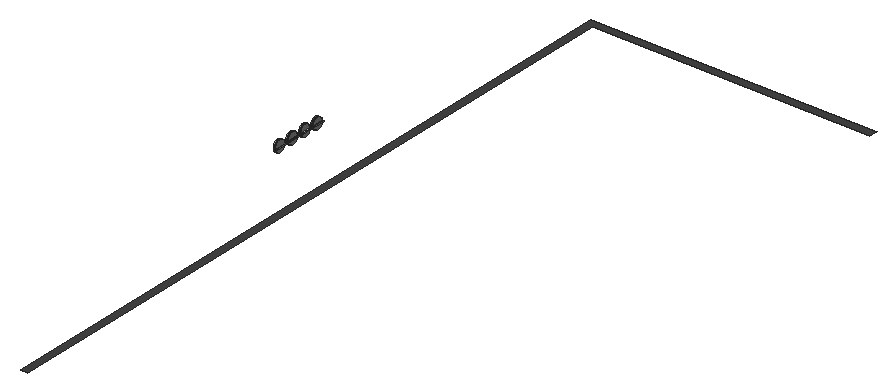
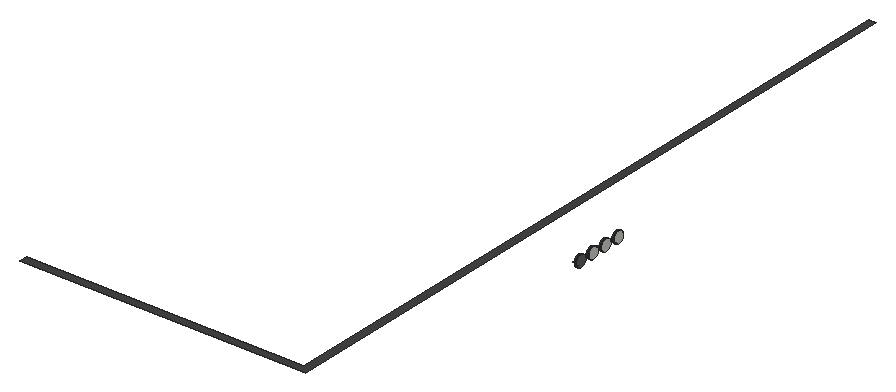
# SketchUp Ruby script. Lengths in inches.
U = 1.inch
M = Sketchup.active_model
def pt(a) = Geom::Point3d.new(a.map { |v| v * U })
def face(e, loops, mat)
  f = e.add_face(loops[0].map { |a| pt(a) })
  loops[1..].each { |l| e.add_face(l.map { |a| pt(a) }).erase! }
  f.material = f.back_material = mat if mat
  f
end
# faces: each face lists its corners as indices into pts; further lists are holes
def faces(e, pts, list, mat = nil) = list.each { |f| face(e, (f[0].is_a?(Array) ? f : [f]).map { |l| l.map { |i| pts[i] } }, mat) }
# xy, xz, yz: faces in a plane at the given z, y or x. An outline is a flat list of corners, or four numbers for a rectangle; further outlines are holes
def ring(l) = l.size == 4 ? [[l[0], l[1]], [l[2], l[1]], [l[2], l[3]], [l[0], l[3]]] : l.each_slice(2).to_a
def flat(e, list, mat, &to3) = list.each { |f| face(e, (f[0].is_a?(Array) ? f : [f]).map { |l| ring(l).map { |u, v| to3.(u, v) } }, mat) }
def xy(e, z, list, mat = nil) = flat(e, list, mat) { |x, y| [x, y, z] }
def xz(e, y, list, mat = nil) = flat(e, list, mat) { |x, z| [x, y, z] }
def yz(e, x, list, mat = nil) = flat(e, list, mat) { |y, z| [x, y, z] }
def lines(e, pts, list) = list.each { |a, b| e.add_line(pt(pts[a]), pt(pts[b])) }
# prism: a flat outline (further loops are holes) pulled along v
def prism(e, loops, v, mat = nil)
  f = face(e, loops, mat); d = Geom::Vector3d.new(v.map { |x| x * U })
  f.pushpull(f.normal.samedirection?(d) ? d.length : -d.length)
end
def box(e, o, s, mat = nil) = prism(e, [[o, [o[0] + s[0], o[1], o[2]], [o[0] + s[0], o[1] + s[1], o[2]], [o[0], o[1] + s[1], o[2]]]], [0, 0, s[2]], mat)
def at(x, y, z, deg = 0) = Geom::Transformation.translation(pt([x, y, z])) * Geom::Transformation.rotation(ORIGIN, Z_AXIS, deg.degrees)
def axes(o, x, y, z) = Geom::Transformation.new([*x, 0, *y, 0, *z, 0, *pt(o).to_a, 1])
def part(name) = M.definitions.add(name)
# library, detail: a bought-in or finely detailed component or shape, given as its bounding box
def library(name, o, s) = part(name).tap { |d| box(d.entities, o, s) }
def detail(e, o, s) = box(e.add_group.entities, o, s)
def put(e, d, t, mat = nil) = e.add_instance(d, t).tap { |i| i.material = mat if mat }
def group(e, t, mat = nil) = e.add_group.tap { |g| g.transformation = t; g.material = mat if mat }.entities
root = M.entities
M.materials.add("[0134_DimGray]").color = [105, 105, 105]
M.materials.add("[Granite Dark Gray]").color = [69, 68, 68]
xy(root,110.72,[[126.73,150.81,127.73,151.02],[126.73,156.81,127.73,157.02],[126.73,162.81,127.73,163.02]],"[0134_DimGray]")
xy(root,111,[[150,0,153,0,153,267,258,267,258,270,150,270]],"[Granite Dark Gray]")
xy(root,112.48,[[127.73,148.85,128.23,152.82],[127.73,154.85,128.23,158.82],[127.73,160.85,128.23,164.82]],"[0134_DimGray]")
xy(root,112.5,[[127.73,166.66,128.23,170.65]],"[0134_DimGray]")
xy(root,112.73,[[127.73,166.66,128.23,170.64]],"[0134_DimGray]")
xy(root,112.74,[[127.73,148.84,128.23,152.82],[127.73,154.84,128.23,158.82],[127.73,160.84,128.23,164.82]],"[0134_DimGray]")
xz(root,148.84,[[126.73,112.53,127.73,112.74],[127.73,112.53,128.23,112.74]],"[0134_DimGray]")
xz(root,152.82,[[127.73,112.48,128.23,112.74]],"[0134_DimGray]")
xz(root,154.84,[[126.73,112.53,127.73,112.74],[127.73,112.53,128.23,112.74]],"[0134_DimGray]")
xz(root,158.82,[[127.73,112.48,128.23,112.74]],"[0134_DimGray]")
xz(root,160.84,[[126.73,112.53,127.73,112.74],[127.73,112.53,128.23,112.74]],"[0134_DimGray]")
xz(root,164.82,[[127.73,112.48,128.23,112.74]])
xz(root,166.66,[[127.73,112.5,128.23,112.73]],"[0134_DimGray]")
xz(root,170.64,[[127.73,112.71,128.23,112.73]],"[0134_DimGray]")
yz(root,126.73,[[150.81,110.72,150.6,110.73,150.39,110.77,150.19,110.82,150,110.9,149.8125,111,149.64,111.11,149.48,111.25,149.33,111.4,149.2,111.5625,149.09,111.74,149,111.93,148.92,112.125,148.875,112.33,148.84,112.53,148.84,112.74,148.85,112.95,148.89,113.16,148.94,113.36,149.02,113.55,149.12,113.74,149.23,113.91,149.37,114.07,149.52,114.22,149.68,114.35,149.86,114.46,150.05,114.55,150.24,114.625,150.45,114.68,150.65,114.71,150.86,114.72,151.07,114.7,151.28,114.67,151.48,114.61,151.67,114.53,151.86,114.43,152.03,114.32,152.19,114.18,152.34,114.03,152.47,113.87,152.58,113.69,152.67,113.5,152.75,113.31,152.8,113.1,152.83,112.9,152.84,112.6875,152.82,112.48,152.79,112.27,152.73,112.07,152.65,111.875,152.55,111.69,152.4375,111.52,152.3,111.36,152.15,111.21,151.99,111.08,151.8125,110.97,151.625,110.875,151.43,110.8,151.22,110.75,151.02,110.72],[156.81,110.72,156.6,110.73,156.39,110.77,156.19,110.82,156,110.9,155.8125,111,155.64,111.11,155.48,111.25,155.33,111.4,155.2,111.5625,155.09,111.74,155,111.93,154.92,112.125,154.875,112.33,154.84,112.53,154.84,112.74,154.85,112.95,154.89,113.16,154.94,113.36,155.02,113.55,155.12,113.74,155.23,113.91,155.37,114.07,155.52,114.22,155.68,114.35,155.86,114.46,156.05,114.55,156.24,114.625,156.45,114.68,156.65,114.71,156.86,114.72,157.07,114.7,157.28,114.67,157.48,114.61,157.67,114.53,157.86,114.43,158.03,114.32,158.19,114.18,158.34,114.03,158.47,113.87,158.58,113.69,158.67,113.5,158.75,113.31,158.8,113.1,158.83,112.9,158.84,112.6875,158.82,112.48,158.79,112.27,158.73,112.07,158.65,111.875,158.55,111.69,158.4375,111.52,158.3,111.36,158.15,111.21,157.99,111.08,157.8125,110.97,157.625,110.875,157.43,110.8,157.22,110.75,157.02,110.72],[162.81,110.72,162.6,110.73,162.39,110.77,162.19,110.82,162,110.9,161.8125,111,161.64,111.11,161.48,111.25,161.33,111.4,161.2,111.5625,161.09,111.74,161,111.93,160.92,112.125,160.875,112.33,160.84,112.53,160.84,112.74,160.85,112.95,160.89,113.16,160.94,113.36,161.02,113.55,161.12,113.74,161.23,113.91,161.37,114.07,161.52,114.22,161.68,114.35,161.86,114.46,162.05,114.55,162.24,114.625,162.45,114.68,162.65,114.71,162.86,114.72,163.07,114.7,163.28,114.67,163.48,114.61,163.67,114.53,163.86,114.43,164.03,114.32,164.19,114.18,164.34,114.03,164.47,113.87,164.58,113.69,164.67,113.5,164.75,113.31,164.8,113.1,164.83,112.9,164.84,112.6875,164.82,112.48,164.79,112.27,164.73,112.07,164.65,111.875,164.55,111.69,164.4375,111.52,164.3,111.36,164.15,111.21,163.99,111.08,163.8125,110.97,163.625,110.875,163.43,110.8,163.22,110.75,163.02,110.72]])
yz(root,126.73,[[168.64,110.51,168.43,110.52,168.23,110.56,168.02,110.61,167.83,110.6875,167.64,110.79,167.47,110.9,167.31,111.03,167.16,111.18,167.03,111.34,166.91,111.52,166.82,111.71,166.75,111.9,166.69,112.11,166.66,112.3125,166.65,112.52,166.66,112.73,166.7,112.9375,166.75,113.14,166.83,113.33,166.92,113.52,167.04,113.7,167.17,113.86,167.32,114.01,167.48,114.14,167.66,114.25,167.85,114.34,168.04,114.42,168.25,114.47,168.45,114.5,168.66,114.51,168.87,114.5,169.08,114.47,169.28,114.41,169.47,114.34,169.66,114.24,169.84,114.125,170,113.99,170.14,113.84,170.28,113.68,170.39,113.5,170.48,113.32,170.56,113.12,170.61,112.92,170.64,112.71,170.65,112.5,170.64,112.29,170.61,112.09,170.55,111.89,170.47,111.69,170.38,111.5,170.26,111.33,170.13,111.17,169.98,111.02,169.82,110.89,169.64,110.78,169.46,110.68,169.26,110.61,169.06,110.55,168.85,110.52]],"[0134_DimGray]")
yz(root,127.73,[[148.84,112.48,148.85,112.48,148.84,112.53,148.84,112.74],[154.85,112.48,154.84,112.53,154.84,112.74,158.82,112.74,158.82,112.48],[160.85,112.48,160.84,112.53,160.84,112.74,164.82,112.74,164.82,112.48],[170.65,112.5,170.65,112.73,170.64,112.73,170.64,112.71]])
yz(root,127.73,[[168.64,110.51,168.85,110.52,169.06,110.55,169.26,110.61,169.46,110.68,169.64,110.78,169.82,110.89,169.98,111.02,170.13,111.17,170.26,111.33,170.38,111.5,170.47,111.69,170.55,111.89,170.61,112.09,170.64,112.29,170.65,112.5,166.66,112.5,166.66,112.73,166.65,112.52,166.66,112.3125,166.69,112.11,166.75,111.9,166.82,111.71,166.91,111.52,167.03,111.34,167.16,111.18,167.31,111.03,167.47,110.9,167.64,110.79,167.83,110.6875,168.02,110.61,168.23,110.56,168.43,110.52],[150.81,110.72,151.02,110.72,151.22,110.75,151.43,110.8,151.625,110.875,151.8125,110.97,151.99,111.08,152.15,111.21,152.3,111.36,152.4375,111.52,152.55,111.69,152.65,111.875,152.73,112.07,152.79,112.27,152.82,112.48,148.85,112.48,148.875,112.33,148.92,112.125,149,111.93,149.09,111.74,149.2,111.5625,149.33,111.4,149.48,111.25,149.64,111.11,149.8125,111,150,110.9,150.19,110.82,150.39,110.77,150.6,110.73],[156.81,110.72,157.02,110.72,157.22,110.75,157.43,110.8,157.625,110.875,157.8125,110.97,157.99,111.08,158.15,111.21,158.3,111.36,158.4375,111.52,158.55,111.69,158.65,111.875,158.73,112.07,158.79,112.27,158.82,112.48,154.85,112.48,154.875,112.33,154.92,112.125,155,111.93,155.09,111.74,155.2,111.5625,155.33,111.4,155.48,111.25,155.64,111.11,155.8125,111,156,110.9,156.19,110.82,156.39,110.77,156.6,110.73],[162.81,110.72,163.02,110.72,163.22,110.75,163.43,110.8,163.625,110.875,163.8125,110.97,163.99,111.08,164.15,111.21,164.3,111.36,164.4375,111.52,164.55,111.69,164.65,111.875,164.73,112.07,164.79,112.27,164.82,112.48,160.85,112.48,160.875,112.33,160.92,112.125,161,111.93,161.09,111.74,161.2,111.5625,161.33,111.4,161.48,111.25,161.64,111.11,161.8125,111,162,110.9,162.19,110.82,162.39,110.77,162.6,110.73],[152.82,112.48,152.84,112.6875,152.83,112.9,152.8,113.1,152.75,113.31,152.67,113.5,152.58,113.69,152.47,113.87,152.34,114.03,152.19,114.18,152.03,114.32,151.86,114.43,151.67,114.53,151.48,114.61,151.28,114.67,151.07,114.7,150.86,114.72,150.65,114.71,150.45,114.68,150.24,114.625,150.05,114.55,149.86,114.46,149.68,114.35,149.52,114.22,149.37,114.07,149.23,113.91,149.12,113.74,149.02,113.55,148.94,113.36,148.89,113.16,148.85,112.95,148.84,112.74,152.82,112.74],
  [158.82,112.48,158.84,112.6875,158.83,112.9,158.8,113.1,158.75,113.31,158.67,113.5,158.58,113.69,158.47,113.87,158.34,114.03,158.19,114.18,158.03,114.32,157.86,114.43,157.67,114.53,157.48,114.61,157.28,114.67,157.07,114.7,156.86,114.72,156.65,114.71,156.45,114.68,156.24,114.625,156.05,114.55,155.86,114.46,155.68,114.35,155.52,114.22,155.37,114.07,155.23,113.91,155.12,113.74,155.02,113.55,154.94,113.36,154.89,113.16,154.85,112.95,154.84,112.74,158.82,112.74],[164.82,112.48,164.84,112.6875,164.83,112.9,164.8,113.1,164.75,113.31,164.67,113.5,164.58,113.69,164.47,113.87,164.34,114.03,164.19,114.18,164.03,114.32,163.86,114.43,163.67,114.53,163.48,114.61,163.28,114.67,163.07,114.7,162.86,114.72,162.65,114.71,162.45,114.68,162.24,114.625,162.05,114.55,161.86,114.46,161.68,114.35,161.52,114.22,161.37,114.07,161.23,113.91,161.12,113.74,161.02,113.55,160.94,113.36,160.89,113.16,160.85,112.95,160.84,112.74,164.82,112.74],[166.66,112.5,166.66,112.73,170.64,112.73,170.64,112.71,170.65,112.5],[166.66,112.73,170.64,112.73,170.61,112.92,170.56,113.12,170.48,113.32,170.39,113.5,170.28,113.68,170.14,113.84,170,113.99,169.84,114.125,169.66,114.24,169.47,114.34,169.28,114.41,169.08,114.47,168.87,114.5,168.66,114.51,168.45,114.5,168.25,114.47,168.04,114.42,167.85,114.34,167.66,114.25,167.48,114.14,167.32,114.01,167.17,113.86,167.04,113.7,166.92,113.52,166.83,113.33,166.75,113.14,166.7,112.9375]],"[0134_DimGray]")
yz(root,128.23,[[148.85,112.48,152.82,112.48,152.82,112.74,148.84,112.74,148.84,112.53],[154.85,112.48,158.82,112.48,158.82,112.74,154.84,112.74,154.84,112.53],[160.85,112.48,164.82,112.48,164.82,112.74,160.84,112.74,160.84,112.53],[166.66,112.5,170.65,112.5,170.64,112.71,170.64,112.73,166.66,112.73]],"[0134_DimGray]")
p = [[126.73,168.23,110.56],[126.73,168.43,110.52],[127.73,168.43,110.52],[127.73,168.23,110.56],[126.73,168.64,110.51],[127.73,168.64,110.51],
  [126.73,168.85,110.52],[127.73,168.85,110.52],[126.73,169.06,110.55],[127.73,169.06,110.55],[126.73,167.83,110.6875],[126.73,168.02,110.61],
  [127.73,168.02,110.61],[127.73,167.83,110.6875],[126.73,169.26,110.61],[127.73,169.26,110.61],[126.73,169.46,110.68],[127.73,169.46,110.68],
  [126.73,150.39,110.77],[126.73,150.6,110.73],[127.73,150.6,110.73],[127.73,150.39,110.77],[126.73,150.81,110.72],[127.73,150.81,110.72],
  [126.73,151.02,110.72],[126.73,151.22,110.75],[127.73,151.22,110.75],[127.73,151.02,110.72],[126.73,156.39,110.77],[126.73,156.6,110.73],
  [127.73,156.6,110.73],[127.73,156.39,110.77],[126.73,156.81,110.72],[127.73,156.81,110.72],[126.73,157.02,110.72],[126.73,157.22,110.75],
  [127.73,157.22,110.75],[127.73,157.02,110.72],[126.73,162.39,110.77],[126.73,162.6,110.73],[127.73,162.6,110.73],[127.73,162.39,110.77],
  [126.73,162.81,110.72],[127.73,162.81,110.72],[126.73,163.02,110.72],[126.73,163.22,110.75],[127.73,163.22,110.75],[127.73,163.02,110.72],
  [126.73,167.64,110.79],[127.73,167.64,110.79],[126.73,169.64,110.78],[127.73,169.64,110.78],[126.73,150,110.9],[126.73,150.19,110.82],
  [127.73,150.19,110.82],[127.73,150,110.9],[126.73,151.43,110.8],[127.73,151.43,110.8],[126.73,151.625,110.875],[127.73,151.625,110.875],
  [126.73,156,110.9],[126.73,156.19,110.82],[127.73,156.19,110.82],[127.73,156,110.9],[126.73,157.43,110.8],[127.73,157.43,110.8],
  [126.73,157.625,110.875],[127.73,157.625,110.875],[126.73,162,110.9],[126.73,162.19,110.82],[127.73,162.19,110.82],[127.73,162,110.9],
  [126.73,163.43,110.8],[127.73,163.43,110.8],[126.73,163.625,110.875],[127.73,163.625,110.875],[126.73,167.47,110.9],[127.73,167.47,110.9],
  [126.73,169.82,110.89],[127.73,169.82,110.89],[126.73,149.8125,111],[127.73,149.8125,111],[126.73,151.8125,110.97],[127.73,151.8125,110.97],
  [126.73,155.8125,111],[127.73,155.8125,111],[126.73,157.8125,110.97],[127.73,157.8125,110.97],[126.73,161.8125,111],[127.73,161.8125,111],
  [126.73,163.8125,110.97],[127.73,163.8125,110.97],[126.73,167.31,111.03],[127.73,167.31,111.03],[126.73,169.98,111.02],[127.73,169.98,111.02],
  [126.73,149.64,111.11],[127.73,149.64,111.11],[126.73,151.99,111.08],[127.73,151.99,111.08],[126.73,155.64,111.11],[127.73,155.64,111.11],
  [126.73,157.99,111.08],[127.73,157.99,111.08],[126.73,161.64,111.11],[127.73,161.64,111.11],[126.73,163.99,111.08],[127.73,163.99,111.08],
  [126.73,167.16,111.18],[127.73,167.16,111.18],[126.73,170.13,111.17],[127.73,170.13,111.17],[126.73,149.48,111.25],[127.73,149.48,111.25],
  [126.73,152.15,111.21],[127.73,152.15,111.21],[126.73,155.48,111.25],[127.73,155.48,111.25],[126.73,158.15,111.21],[127.73,158.15,111.21],
  [126.73,161.48,111.25],[127.73,161.48,111.25],[126.73,164.15,111.21],[127.73,164.15,111.21],[126.73,149.33,111.4],[127.73,149.33,111.4],
  [126.73,152.3,111.36],[127.73,152.3,111.36],[126.73,155.33,111.4],[127.73,155.33,111.4],[126.73,158.3,111.36],[127.73,158.3,111.36],
  [126.73,161.33,111.4],[127.73,161.33,111.4],[126.73,164.3,111.36],[127.73,164.3,111.36],[126.73,167.03,111.34],[127.73,167.03,111.34],
  [126.73,170.26,111.33],[127.73,170.26,111.33],[126.73,166.91,111.52],[127.73,166.91,111.52],[126.73,170.38,111.5],[127.73,170.38,111.5],
  [126.73,149.2,111.5625],[127.73,149.2,111.5625],[126.73,152.4375,111.52],[127.73,152.4375,111.52],[126.73,155.2,111.5625],[127.73,155.2,111.5625],
  [126.73,158.4375,111.52],[127.73,158.4375,111.52],[126.73,161.2,111.5625],[127.73,161.2,111.5625],[126.73,164.4375,111.52],[127.73,164.4375,111.52],
  [126.73,152.55,111.69],[127.73,152.55,111.69],[126.73,158.55,111.69],[127.73,158.55,111.69],[126.73,164.55,111.69],[127.73,164.55,111.69],
  [126.73,166.82,111.71],[127.73,166.82,111.71],[126.73,170.47,111.69],[127.73,170.47,111.69],[126.73,149.09,111.74],[127.73,149.09,111.74],
  [126.73,155.09,111.74],[127.73,155.09,111.74],[126.73,161.09,111.74],[127.73,161.09,111.74],[126.73,149,111.93],[127.73,149,111.93],
  [126.73,152.65,111.875],[127.73,152.65,111.875],[126.73,155,111.93],[127.73,155,111.93],[126.73,158.65,111.875],[127.73,158.65,111.875],
  [126.73,161,111.93],[127.73,161,111.93],[126.73,164.65,111.875],[127.73,164.65,111.875],[126.73,166.75,111.9],[127.73,166.75,111.9],
  [126.73,170.55,111.89],[127.73,170.55,111.89],[126.73,148.92,112.125],[127.73,148.92,112.125],[126.73,152.73,112.07],[127.73,152.73,112.07],
  [126.73,154.92,112.125],[127.73,154.92,112.125],[126.73,158.73,112.07],[127.73,158.73,112.07],[126.73,160.92,112.125],[127.73,160.92,112.125],
  [126.73,164.73,112.07],[127.73,164.73,112.07],[126.73,166.69,112.11],[127.73,166.69,112.11],[126.73,170.61,112.09],[127.73,170.61,112.09],
  [126.73,148.875,112.33],[127.73,148.875,112.33],[126.73,152.79,112.27],[127.73,152.79,112.27],[126.73,154.875,112.33],[127.73,154.875,112.33],
  [126.73,158.79,112.27],[127.73,158.79,112.27],[126.73,160.875,112.33],[127.73,160.875,112.33],[126.73,164.79,112.27],[127.73,164.79,112.27],
  [126.73,166.66,112.3125],[127.73,166.66,112.3125],[126.73,170.64,112.29],[127.73,170.64,112.29],[126.73,148.84,112.53],[127.73,148.85,112.48],
  [127.73,148.84,112.53],[126.73,152.82,112.48],[127.73,152.82,112.48],[126.73,154.84,112.53],[127.73,154.85,112.48],[127.73,154.84,112.53],
  [126.73,158.82,112.48],[127.73,158.82,112.48],[126.73,160.84,112.53],[127.73,160.85,112.48],[127.73,160.84,112.53],[126.73,164.82,112.48],
  [127.73,164.82,112.48],[126.73,166.65,112.52],[127.73,166.65,112.52],[126.73,170.65,112.5],[127.73,170.65,112.5],[128.23,148.85,112.48],
  [128.23,148.84,112.53],[126.73,152.84,112.6875],[127.73,152.84,112.6875],[128.23,154.85,112.48],[128.23,154.84,112.53],[126.73,158.84,112.6875],
  [127.73,158.84,112.6875],[128.23,160.85,112.48],[128.23,160.84,112.53],[126.73,164.84,112.6875],[127.73,164.84,112.6875],[126.73,166.66,112.73],
  [127.73,166.66,112.73],[126.73,170.64,112.71],[127.73,170.64,112.71],[128.23,170.64,112.71],[128.23,170.65,112.5],[126.73,148.85,112.95],
  [126.73,148.84,112.74],[127.73,148.84,112.74],[127.73,148.85,112.95],[126.73,152.83,112.9],[127.73,152.83,112.9],[126.73,154.85,112.95],
  [126.73,154.84,112.74],[127.73,154.84,112.74],[127.73,154.85,112.95],[126.73,158.83,112.9],[127.73,158.83,112.9],[126.73,160.85,112.95],
  [126.73,160.84,112.74],[127.73,160.84,112.74],[127.73,160.85,112.95],[126.73,164.83,112.9],[127.73,164.83,112.9],[126.73,166.7,112.9375],
  [127.73,166.7,112.9375],[126.73,170.61,112.92],[127.73,170.61,112.92],[127.73,170.64,112.73],[126.73,152.8,113.1],[127.73,152.8,113.1],
  [126.73,158.8,113.1],[127.73,158.8,113.1],[126.73,164.8,113.1],[127.73,164.8,113.1],[126.73,166.75,113.14],[127.73,166.75,113.14],
  [126.73,170.56,113.12],[127.73,170.56,113.12],[126.73,148.89,113.16],[127.73,148.89,113.16],[126.73,154.89,113.16],[127.73,154.89,113.16],
  [126.73,160.89,113.16],[127.73,160.89,113.16],[126.73,152.75,113.31],[127.73,152.75,113.31],[126.73,158.75,113.31],[127.73,158.75,113.31],
  [126.73,164.75,113.31],[127.73,164.75,113.31],[126.73,166.83,113.33],[127.73,166.83,113.33],[126.73,170.48,113.32],[127.73,170.48,113.32],
  [126.73,148.94,113.36],[127.73,148.94,113.36],[126.73,154.94,113.36],[127.73,154.94,113.36],[126.73,160.94,113.36],[127.73,160.94,113.36],
  [126.73,152.67,113.5],[127.73,152.67,113.5],[126.73,158.67,113.5],[127.73,158.67,113.5],[126.73,164.67,113.5],[127.73,164.67,113.5],
  [126.73,166.92,113.52],[127.73,166.92,113.52],[126.73,170.39,113.5],[127.73,170.39,113.5],[126.73,149.02,113.55],[127.73,149.02,113.55],
  [126.73,155.02,113.55],[127.73,155.02,113.55],[126.73,161.02,113.55],[127.73,161.02,113.55],[126.73,152.58,113.69],[127.73,152.58,113.69],
  [126.73,158.58,113.69],[127.73,158.58,113.69],[126.73,164.58,113.69],[127.73,164.58,113.69],[126.73,167.04,113.7],[127.73,167.04,113.7],
  [126.73,170.28,113.68],[127.73,170.28,113.68],[126.73,149.12,113.74],[127.73,149.12,113.74],[126.73,155.12,113.74],[127.73,155.12,113.74],
  [126.73,161.12,113.74],[127.73,161.12,113.74],[126.73,149.23,113.91],[127.73,149.23,113.91],[126.73,152.47,113.87],[127.73,152.47,113.87],
  [126.73,155.23,113.91],[127.73,155.23,113.91],[126.73,158.47,113.87],[127.73,158.47,113.87],[126.73,161.23,113.91],[127.73,161.23,113.91],
  [126.73,164.47,113.87],[127.73,164.47,113.87],[126.73,167.17,113.86],[127.73,167.17,113.86],[126.73,170.14,113.84],[127.73,170.14,113.84],
  [126.73,170,113.99],[127.73,170,113.99],[126.73,149.37,114.07],[127.73,149.37,114.07],[126.73,152.34,114.03],[127.73,152.34,114.03],
  [126.73,155.37,114.07],[127.73,155.37,114.07],[126.73,158.34,114.03],[127.73,158.34,114.03],[126.73,161.37,114.07],[127.73,161.37,114.07],
  [126.73,164.34,114.03],[127.73,164.34,114.03],[126.73,167.32,114.01],[127.73,167.32,114.01],[126.73,152.19,114.18],[127.73,152.19,114.18],
  [126.73,158.19,114.18],[127.73,158.19,114.18],[126.73,164.19,114.18],[127.73,164.19,114.18],[126.73,167.48,114.14],[127.73,167.48,114.14],
  [126.73,169.84,114.125],[127.73,169.84,114.125],[126.73,149.52,114.22],[127.73,149.52,114.22],[126.73,155.52,114.22],[127.73,155.52,114.22],
  [126.73,161.52,114.22],[127.73,161.52,114.22],[126.73,167.66,114.25],[127.73,167.66,114.25],[126.73,169.66,114.24],[127.73,169.66,114.24],
  [126.73,149.68,114.35],[127.73,149.68,114.35],[126.73,152.03,114.32],[127.73,152.03,114.32],[126.73,155.68,114.35],[127.73,155.68,114.35],
  [126.73,158.03,114.32],[127.73,158.03,114.32],[126.73,161.68,114.35],[127.73,161.68,114.35],[126.73,164.03,114.32],[127.73,164.03,114.32],
  [126.73,167.85,114.34],[127.73,167.85,114.34],[126.73,169.47,114.34],[127.73,169.47,114.34],[126.73,149.86,114.46],[127.73,149.86,114.46],
  [126.73,151.86,114.43],[127.73,151.86,114.43],[126.73,155.86,114.46],[127.73,155.86,114.46],[126.73,157.86,114.43],[127.73,157.86,114.43],
  [126.73,161.86,114.46],[127.73,161.86,114.46],[126.73,163.86,114.43],[127.73,163.86,114.43],[126.73,168.04,114.42],[127.73,168.04,114.42],
  [126.73,169.28,114.41],[127.73,169.28,114.41],[126.73,151.67,114.53],[127.73,151.67,114.53],[126.73,157.67,114.53],[127.73,157.67,114.53],
  [126.73,163.67,114.53],[127.73,163.67,114.53],[126.73,168.25,114.47],[127.73,168.25,114.47],[126.73,169.08,114.47],[127.73,169.08,114.47],
  [126.73,150.05,114.55],[127.73,150.05,114.55],[126.73,151.48,114.61],[127.73,151.48,114.61],[126.73,156.05,114.55],[127.73,156.05,114.55],
  [126.73,157.48,114.61],[127.73,157.48,114.61],[126.73,162.05,114.55],[127.73,162.05,114.55],[126.73,163.48,114.61],[127.73,163.48,114.61],
  [126.73,168.45,114.5],[127.73,168.45,114.5],[126.73,168.66,114.51],[127.73,168.66,114.51],[126.73,168.87,114.5],[127.73,168.87,114.5],
  [126.73,150.24,114.625],[127.73,150.24,114.625],[126.73,150.45,114.68],[127.73,150.45,114.68],[126.73,151.28,114.67],[127.73,151.28,114.67],
  [126.73,156.24,114.625],[127.73,156.24,114.625],[126.73,156.45,114.68],[127.73,156.45,114.68],[126.73,157.28,114.67],[127.73,157.28,114.67],
  [126.73,162.24,114.625],[127.73,162.24,114.625],[126.73,162.45,114.68],[127.73,162.45,114.68],[126.73,163.28,114.67],[127.73,163.28,114.67],
  [126.73,150.65,114.71],[127.73,150.65,114.71],[126.73,150.86,114.72],[127.73,150.86,114.72],[126.73,151.07,114.7],[127.73,151.07,114.7],
  [126.73,156.65,114.71],[127.73,156.65,114.71],[126.73,156.86,114.72],[127.73,156.86,114.72],[126.73,157.07,114.7],[127.73,157.07,114.7],
  [126.73,162.65,114.71],[127.73,162.65,114.71],[126.73,162.86,114.72],[127.73,162.86,114.72],[126.73,163.07,114.7],[127.73,163.07,114.7]]
faces(root,p,[[0,1,2,3],[1,4,5,2],[4,6,7,5],[6,8,9,7],[10,11,12,13],[11,0,3,12],[8,14,15,9],[14,16,17,15],
  [18,19,20,21],[19,22,23,20],[24,25,26,27],[28,29,30,31],[29,32,33,30],[34,35,36,37],[38,39,40,41],[39,42,43,40],
  [44,45,46,47],[48,10,13,49],[16,50,51,17],[52,53,54,55],[53,18,21,54],[25,56,57,26],[56,58,59,57],[60,61,62,63],
  [61,28,31,62],[35,64,65,36],[64,66,67,65],[68,69,70,71],[69,38,41,70],[45,72,73,46],[72,74,75,73],[76,48,49,77],
  [50,78,79,51],[80,52,55,81],[58,82,83,59],[84,60,63,85],[66,86,87,67],[88,68,71,89],[74,90,91,75],[92,76,77,93],
  [78,94,95,79],[96,80,81,97],[82,98,99,83],[100,84,85,101],[86,102,103,87],[104,88,89,105],[90,106,107,91],[108,92,93,109],
  [94,110,111,95],[112,96,97,113],[98,114,115,99],[116,100,101,117],[102,118,119,103],[120,104,105,121],[106,122,123,107],[124,112,113,125],
  [114,126,127,115],[128,116,117,129],[118,130,131,119],[132,120,121,133],[122,134,135,123],[136,108,109,137],[110,138,139,111],[140,136,137,141],
  [138,142,143,139],[144,124,125,145],[126,146,147,127],[148,128,129,149],[130,150,151,131],[152,132,133,153],[134,154,155,135],[146,156,157,147],
  [150,158,159,151],[154,160,161,155],[162,140,141,163],[142,164,165,143],[166,144,145,167],[168,148,149,169],[170,152,153,171],[172,166,167,173],
  [156,174,175,157],[176,168,169,177],[158,178,179,159],[180,170,171,181],[160,182,183,161],[184,162,163,185],[164,186,187,165],[188,172,173,189],
  [174,190,191,175],[192,176,177,193],[178,194,195,179],[196,180,181,197],[182,198,199,183],[200,184,185,201],[186,202,203,187],[204,188,189,205],
  [190,206,207,191],[208,192,193,209],[194,210,211,195],[212,196,197,213],[198,214,215,199],[216,200,201,217],[202,218,219,203],[220,204,205,221,222],
  [206,223,224,207],[225,208,209,226,227],[210,228,229,211],[230,212,213,231,232],[214,233,234,215],[235,216,217,236],[218,237,238,219],[222,221,239,240],
  [223,241,242,224],[227,226,243,244],[228,245,246,229],[232,231,247,248],[233,249,250,234],[251,235,236,252],[237,253,254,238],[238,254,255,256],
  [257,258,259,260],[241,261,262,242],[263,264,265,266],[245,267,268,246],[269,270,271,272],[249,273,274,250],[275,251,252,276],[253,277,278,279,254],
  [261,280,281,262],[267,282,283,268],[273,284,285,274],[286,275,276,287],[277,288,289,278],[290,257,260,291],[292,263,266,293],[294,269,272,295],
  [280,296,297,281],[282,298,299,283],[284,300,301,285],[302,286,287,303],[288,304,305,289],[306,290,291,307],[308,292,293,309],[310,294,295,311],
  [296,312,313,297],[298,314,315,299],[300,316,317,301],[318,302,303,319],[304,320,321,305],[322,306,307,323],[324,308,309,325],[326,310,311,327],
  [312,328,329,313],[314,330,331,315],[316,332,333,317],[334,318,319,335],[320,336,337,321],[338,322,323,339],[340,324,325,341],[342,326,327,343],
  [344,338,339,345],[328,346,347,329],[348,340,341,349],[330,350,351,331],[352,342,343,353],[332,354,355,333],[356,334,335,357],[336,358,359,337],
  [358,360,361,359],[362,344,345,363],[346,364,365,347],[366,348,349,367],[350,368,369,351],[370,352,353,371],[354,372,373,355],[374,356,357,375],
  [364,376,377,365],[368,378,379,369],[372,380,381,373],[382,374,375,383],[360,384,385,361],[386,362,363,387],[388,366,367,389],[390,370,371,391],
  [392,382,383,393],[384,394,395,385],[396,386,387,397],[376,398,399,377],[400,388,389,401],[378,402,403,379],[404,390,391,405],[380,406,407,381],
  [408,392,393,409],[394,410,411,395],[412,396,397,413],[398,414,415,399],[416,400,401,417],[402,418,419,403],[420,404,405,421],[406,422,423,407],
  [424,408,409,425],[410,426,427,411],[414,428,429,415],[418,430,431,419],[422,432,433,423],[434,424,425,435],[426,436,437,427],[438,412,413,439],
  [428,440,441,429],[442,416,417,443],[430,444,445,431],[446,420,421,447],[432,448,449,433],[450,434,435,451],[452,450,451,453],[454,452,453,455],
  [436,454,455,437],[456,438,439,457],[458,456,457,459],[440,460,461,441],[462,442,443,463],[464,462,463,465],[444,466,467,445],[468,446,447,469],
  [470,468,469,471],[448,472,473,449],[474,458,459,475],[476,474,475,477],[478,476,477,479],[460,478,479,461],[480,464,465,481],[482,480,481,483],
  [484,482,483,485],[466,484,485,467],[486,470,471,487],[488,486,487,489],[490,488,489,491],[472,490,491,473]],"[0134_DimGray]")
